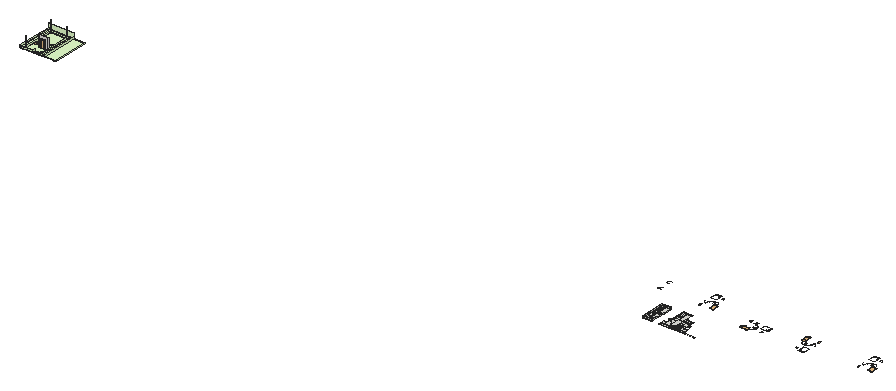
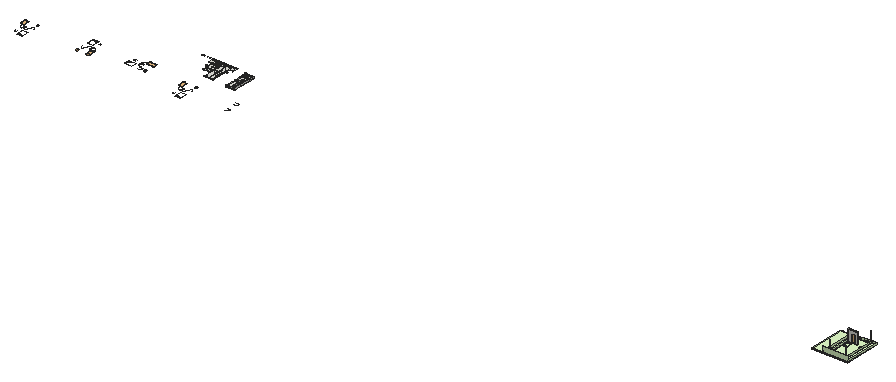
# SketchUp Ruby script. Lengths in inches.
U = 1.inch
M = Sketchup.active_model
def pt(a) = Geom::Point3d.new(a.map { |v| v * U })
def face(e, loops, mat)
  f = e.add_face(loops[0].map { |a| pt(a) })
  loops[1..].each { |l| e.add_face(l.map { |a| pt(a) }).erase! }
  f.material = f.back_material = mat if mat
  f
end
# faces: each face lists its corners as indices into pts; further lists are holes
def faces(e, pts, list, mat = nil) = list.each { |f| face(e, (f[0].is_a?(Array) ? f : [f]).map { |l| l.map { |i| pts[i] } }, mat) }
# xy, xz, yz: faces in a plane at the given z, y or x. An outline is a flat list of corners, or four numbers for a rectangle; further outlines are holes
def ring(l) = l.size == 4 ? [[l[0], l[1]], [l[2], l[1]], [l[2], l[3]], [l[0], l[3]]] : l.each_slice(2).to_a
def flat(e, list, mat, &to3) = list.each { |f| face(e, (f[0].is_a?(Array) ? f : [f]).map { |l| ring(l).map { |u, v| to3.(u, v) } }, mat) }
def xy(e, z, list, mat = nil) = flat(e, list, mat) { |x, y| [x, y, z] }
def xz(e, y, list, mat = nil) = flat(e, list, mat) { |x, z| [x, y, z] }
def yz(e, x, list, mat = nil) = flat(e, list, mat) { |y, z| [x, y, z] }
def lines(e, pts, list) = list.each { |a, b| e.add_line(pt(pts[a]), pt(pts[b])) }
# prism: a flat outline (further loops are holes) pulled along v
def prism(e, loops, v, mat = nil)
  f = face(e, loops, mat); d = Geom::Vector3d.new(v.map { |x| x * U })
  f.pushpull(f.normal.samedirection?(d) ? d.length : -d.length)
end
def box(e, o, s, mat = nil) = prism(e, [[o, [o[0] + s[0], o[1], o[2]], [o[0] + s[0], o[1] + s[1], o[2]], [o[0], o[1] + s[1], o[2]]]], [0, 0, s[2]], mat)
def at(x, y, z, deg = 0) = Geom::Transformation.translation(pt([x, y, z])) * Geom::Transformation.rotation(ORIGIN, Z_AXIS, deg.degrees)
def axes(o, x, y, z) = Geom::Transformation.new([*x, 0, *y, 0, *z, 0, *pt(o).to_a, 1])
def part(name) = M.definitions.add(name)
# library, detail: a bought-in or finely detailed component or shape, given as its bounding box
def library(name, o, s) = part(name).tap { |d| box(d.entities, o, s) }
def detail(e, o, s) = box(e.add_group.entities, o, s)
def put(e, d, t, mat = nil) = e.add_instance(d, t).tap { |i| i.material = mat if mat }
def group(e, t, mat = nil) = e.add_group.tap { |g| g.transformation = t; g.material = mat if mat }.entities
root = M.entities
M.materials.add("[Color F01]").color = [229, 255, 204]
M.materials.add("[Wood Cherry Original]").color = [152, 86, 42]
c1 = part("*U16\#1")
p = [[-20,-17,0],[-20,23,0],[-18.25,23,0],[-18.25,-17,0],[20,-17,0],[19.92,-14.49,0],
  [19.68,-11.99,0],[19.29,-9.5,0],[18.74,-7.05,0],[18.04,-4.64,0],[17.19,-2.28,0],[16.19,0.03,0],
  [15.05,2.27,0],[13.77,4.43,0],[12.36,6.51,0],[10.82,8.5,0],[9.16,10.38,0],[7.38,12.16,0],
  [5.5,13.82,0],[3.51,15.36,0],[1.43,16.77,0],[-0.73,18.05,0],[-2.97,19.19,0],[-5.28,20.19,0],
  [-7.64,21.04,0],[-10.05,21.74,0],[-12.5,22.29,0],[-14.99,22.68,0],[-17.49,22.92,0],[-20,-23,0],
  [20,-23,0]]
lines(c1.entities,p,[[0,1],[1,2],[2,3],[3,0],[4,5],[5,6],[6,7],[7,8],[8,9],[9,10],[10,11],[11,12],
  [12,13],[13,14],[14,15],[15,16],[16,17],[17,18],[18,19],[19,20],[20,21],[21,22],[22,23],[23,24],
  [24,25],[25,26],[26,27],[27,28],[28,1],[0,29],[4,30]])
c2 = part("Bed - Queen\#1")
p = [[22,23.6,0],[16.8,23.6,0],[22,38.8,0],[1.2,38.8,0],[1.2,25.6,0],[-1.2,38.8,0],
  [-1.2,25.6,0],[-22,38.8,0],[-22,25.6,0],[30,-40,0],[-30,-40,0],[-30,40,0],
  [14.8,23.2,0],[-30,23.2,0],[-30,25.6,0],[14.8,25.6,0],[30,40,0],[30,10.4,0],
  [14.8,10.4,0]]
lines(c2.entities,p,[[0,1],[2,0],[3,2],[4,3],[5,6],[7,5],[8,7],[9,10],[10,11],[12,13],[14,15],[11,16],
  [16,9],[17,15],[18,17],[15,18]])
c3 = library("Dining Set - 36 x 72 in.\#1",[-45.5,-27.5,0],[91,55,0.01])
c4 = library("*U20\#1",[-21.75,-46.5,0],[21,33,0.01])
c5 = part("Bed - Queen\#2")
p = [[22,23.6,0],[16.8,23.6,0],[22,38.8,0],[1.2,38.8,0],[1.2,25.6,0],[-1.2,38.8,0],
  [-1.2,25.6,0],[-22,38.8,0],[-22,25.6,0],[30,-40,0],[-30,-40,0],[-30,40,0],
  [14.8,23.2,0],[-30,23.2,0],[-30,25.6,0],[14.8,25.6,0],[30,40,0],[30,10.4,0],
  [14.8,10.4,0]]
lines(c5.entities,p,[[0,1],[2,0],[3,2],[4,3],[5,6],[7,5],[8,7],[9,10],[10,11],[12,13],[14,15],[11,16],
  [16,9],[17,15],[18,17],[15,18]])
c6 = part("*U16\#2")
p = [[-20,-17,0],[-20,23,0],[-18.25,23,0],[-18.25,-17,0],[20,-17,0],[19.92,-14.49,0],
  [19.68,-11.99,0],[19.29,-9.5,0],[18.74,-7.05,0],[18.04,-4.64,0],[17.19,-2.28,0],[16.19,0.03,0],
  [15.05,2.27,0],[13.77,4.43,0],[12.36,6.51,0],[10.82,8.5,0],[9.16,10.38,0],[7.38,12.16,0],
  [5.5,13.82,0],[3.51,15.36,0],[1.43,16.77,0],[-0.73,18.05,0],[-2.97,19.19,0],[-5.28,20.19,0],
  [-7.64,21.04,0],[-10.05,21.74,0],[-12.5,22.29,0],[-14.99,22.68,0],[-17.49,22.92,0],[-20,-23,0],
  [20,-23,0]]
lines(c6.entities,p,[[0,1],[1,2],[2,3],[3,0],[4,5],[5,6],[6,7],[7,8],[8,9],[9,10],[10,11],[11,12],
  [12,13],[13,14],[14,15],[15,16],[16,17],[17,18],[18,19],[19,20],[20,21],[21,22],[22,23],[23,24],
  [24,25],[25,26],[26,27],[27,28],[28,1],[0,29],[4,30]])
c7 = library("Dining Set - 36 x 72 in.\#2",[-45.5,-27.5,0],[91,55,0.01])
c8 = library("*U20\#2",[-21.75,-46.5,0],[21,33,0.01])
c9 = part("Group\#16")
xy(c9.entities,0,[[8.74,0,9,0,9,0.26],[140,3.98,140.02,4,140,4],[0,123.84,0.16,124,0,124],[0,335.97,0.03,336,0,336]])
# 113 loose lines left out
c10 = part("Group\#15")
box(c10.entities,[0,0,0],[67,6,6])
c11 = library("Group\#19",[0,0,0],[36,2,84])
c12 = part("Difference")
prism(c12.entities,[[[0,0,0],[29,0,0],[29,0,84],[65,0,84],[65,0,0],[101,0,0],[101,0,120],[0,0,120]]],[0,10,0])
xy(root,0,[[7085,0,7347,3],[7347,0,7464.37,3],[7085,3,7221,21],[7221,3,7288,9],[7288,3,7347,21],
  [7221,9,7288,15],[7221,15,7288,21],[7085,21,7089,63],[7089,21,7125,63],[7125,21,7221,21,7221,27,7129,27,7129,273,7221,273,7221.38,273.02,7221.76,273.1,7221.95,273.15,7222.125,273.22,7222.3,273.3,7222.47,273.39,7222.64,273.49,7222.79,273.6,7223.09,273.84,7223.22,273.98,7223.35,274.13,7223.46,274.28,7223.57,274.44,7223.66,274.61,7223.74,274.79,7223.82,274.96,7223.875,275.15,7223.92,275.33,7223.96,275.52,7223.99,275.71,7224,275.9,7224,276.1,7223.99,276.29,7223.96,276.48,7223.92,276.67,7223.875,276.85,7223.82,277.04,7223.74,277.21,7223.66,277.39,7223.57,277.56,7223.46,277.72,7223.35,277.87,7223.22,278.02,7223.09,278.16,7222.79,278.4,7222.64,278.51,7222.47,278.61,7222.3,278.7,7222.125,278.78,7221.95,278.85,7221.76,278.9,7221.38,278.98,7221,279,7125,279],
  [7221,21,7307,27],[7307,21,7343,63],[7343,21,7347,63],[7129,27,7221,27,7221,85.4,7218,85.4,7218,62.89,7214.08,61.43,7210.07,60.24,7206,59.31,7201.87,58.64,7197.71,58.24,7193.53,58.11,7189.36,58.26,7185.2,58.67,7181.07,59.36,7177,60.3,7173,61.51,7169.6,62.85,7166.28,64.39,7163.07,66.14,7159.97,68.08,7157,70.21,7154.17,72.52,7151.49,75.01,7148.97,77.66,7146.61,80.45,7144.44,83.39,7142.45,86.46,7142.18,86.94,7140.66,89.65,7139.07,92.9375,7137.6875,96.32,7136.52,99.79,7135.57,103.32,7134.88,106.69,7134.84,106.9,7134.33,110.52,7134.05,114.16,7134,117.82,7134,273,7129,273],[[7221,27,7288,85.4],[7256.5,30,7285,82.4],[7239.51,37.02,7239.51,40.7,7224,40.7,7224,82.4,7252.5,82.4,7252.5,42.7,7247.66,42.7,7247.66,37.02]],
  [7288,27,7307,27,7307,147,7305,147,7305,91.16,7304.96,90.87,7304.91,90.58,7304.83,90.29,7304.74,90.01,7304.63,89.73,7304.5,89.46,7304.36,89.2,7304.2,88.95,7304.02,88.72,7303.83,88.49,7303.625,88.27,7303.41,88.07,7303.18,87.89,7302.93,87.72,7302.68,87.5625,7302.42,87.42,7302.14,87.3,7301.87,87.2,7301.58,87.11,7301.29,87.05,7301,87,7289.57,87,7289.33,86.94,7289.21,86.9,7289.09,86.85,7288.87,86.73,7288.77,86.66,7288.67,86.58,7288.4,86.31,7288.33,86.21,7288.26,86.1,7288.14,85.88,7288.02,85.52,7288,85.4],[7256.5,30,7285,30,7285,40.7,7269.49,40.7,7269.49,37.02,7261.34,37.02,7261.34,40.7,7256.5,40.7],[7239.51,37.02,7247.66,75.22],[7261.34,37.02,7269.49,75.22],[7261.34,37.02,7269.49,75.22],
  [7224,40.7,7239.51,42.7],[7256.5,40.7,7261.34,42.7],[7269.49,40.7,7285,42.7],[7224,42.7,7239.51,55.2],[7247.66,42.7,7252.5,55.2],
  [7256.5,42.7,7261.34,55.2],[7269.49,42.7,7285,55.2],[7224,55.2,7239.51,57.2],[7247.66,55.2,7252.5,57.2],[7256.5,55.2,7261.34,57.2],
  [7269.49,55.2,7285,57.2],[7224,57.2,7239.51,69.7],[7247.66,57.2,7252.5,69.7],[7256.5,57.2,7261.34,69.7],[7269.49,57.2,7285,69.7],
  [7193.53,58.11,7197.71,58.24,7201.87,58.64,7206,59.31,7210.07,60.24,7214.08,61.43,7218,62.89,7218,85.4,7221,85.4,7221,147,7177,147,7177,60.3,7181.07,59.36,7185.2,58.67,7189.36,58.26],[7177,60.3,7177,270,7173,270,7173,61.51],[[7173,61.51,7173,270,7170,270,7170,200.6,7146,200.6,7146,270,7134,270,7134,117.82,7134.05,114.16,7134.33,110.52,7134.84,106.9,7134.88,106.69,7135.57,103.32,7136.52,99.79,7137.6875,96.32,7139.07,92.9375,7140.66,89.65,7142.18,86.94,7142.45,86.46,7144.44,83.39,7146.61,80.45,7148.97,77.66,7151.49,75.01,7154.17,72.52,7157,70.21,7159.97,68.08,7163.07,66.14,7166.28,64.39,7169.6,62.85],[7164.9,119.64,7163.62,119.72,7162.35,119.89,7161.09,120.14,7159.85,120.48,7158.63,120.89,7157.45,121.38,7156.3,121.95,7155.1875,122.59,7154.12,123.3,7153.1,124.09,7152.13,124.93,7151.23,125.84,7150.38,126.8,7149.6,127.82,7148.88,128.89,7148.24,130,7147.67,131.15,7147.17,132.33,7146.76,133.55,7146.61,134.08,7146.42,134.79,7146.17,136.05,7146,137.32,7146,197.6,7170,197.6,7170,120.13,7168.74,119.89,7167.47,119.72,7166.1875,119.64]],[7224,69.7,7239.51,71.7],[7247.66,69.7,7252.5,71.7],
  [7256.5,69.7,7261.34,71.7],[7269.49,69.7,7285,71.7],[7224,71.7,7239.51,71.7,7239.51,75.22,7247.66,75.22,7247.66,71.7,7252.5,71.7,7252.5,82.4,7224,82.4],[7256.5,71.7,7261.34,71.7,7261.34,75.22,7269.49,75.22,7269.49,71.7,7285,71.7,7285,82.4,7256.5,82.4],[7221,85.4,7224.97,85.4,7224.97,115,7269,115,7269,85.4,7288,85.4,7288.02,85.52,7288.14,85.88,7288.26,86.1,7288.33,86.21,7288.4,86.31,7288.67,86.58,7288.77,86.66,7288.87,86.73,7289.09,86.85,7289.21,86.9,7289.33,86.94,7289.57,87,7301,87,7301,147,7221,147],
  [7224.97,85.4,7228.97,85.4,7228.97,111,7265,111,7265,85.4,7269,85.4,7269,115,7224.97,115],[7228.97,85.4,7244.98,111],[7244.98,85.4,7248.98,111],[7248.98,85.4,7265,111],[7301,87,7301.29,87.05,7301.58,87.11,7301.87,87.2,7302.14,87.3,7302.42,87.42,7302.68,87.5625,7302.93,87.72,7303.18,87.89,7303.41,88.07,7303.625,88.27,7303.83,88.49,7304.02,88.72,7304.2,88.95,7304.36,89.2,7304.5,89.46,7304.63,89.73,7304.74,90.01,7304.83,90.29,7304.91,90.58,7304.96,90.87,7305,91.16,7305,147,7301,147],
  [7101,111,7125,115],[7307,111,7331,115],[7164.9,119.64,7166.1875,119.64,7167.47,119.72,7168.74,119.89,7170,120.13,7170,197.6,7146,197.6,7146,137.32,7146.17,136.05,7146.42,134.79,7146.61,134.08,7146.76,133.55,7147.17,132.33,7147.67,131.15,7148.24,130,7148.88,128.89,7149.6,127.82,7150.38,126.8,7151.23,125.84,7152.13,124.93,7153.1,124.09,7154.12,123.3,7155.1875,122.59,7156.3,121.95,7157.45,121.38,7158.63,120.89,7159.85,120.48,7161.09,120.14,7162.35,119.89,7163.62,119.72],[7177,147,7221,153],[7221,147,7307,147,7307.38,147.02,7307.76,147.1,7307.95,147.15,7308.125,147.22,7308.3,147.3,7308.47,147.39,7308.64,147.49,7308.79,147.6,7309.09,147.84,7309.22,147.98,7309.35,148.13,7309.46,148.28,7309.57,148.44,7309.66,148.61,7309.74,148.79,7309.82,148.96,7309.875,149.15,7309.92,149.33,7309.96,149.52,7309.99,149.71,7310,149.9,7310,150.1,7309.99,150.29,7309.96,150.48,7309.92,150.67,7309.875,150.85,7309.82,151.04,7309.74,151.21,7309.66,151.39,7309.57,151.56,7309.46,151.72,7309.35,151.87,7309.22,152.02,7309.09,152.16,7308.79,152.4,7308.64,152.51,7308.47,152.61,7308.3,152.7,7308.125,152.78,7307.95,152.85,7307.76,152.9,7307.38,152.98,7307,153,7221,153],
  [7177,153,7221,156],[7221,153,7305,156],[7177,156,7221,270],[7221,156,7305,158],[7221,158,7244.77,189],
  [7244.77,158,7245.77,189],[7245.77,158,7270.55,189],[7270.55,158,7271.55,189],[7271.55,158,7295,189],[7295,158,7305,189],
  [7221,189,7305,191],[7146,200.6,7170,270],[7134,270,7221,273]])
xy(root,0,[[0,344.07,4,730.07],[4,344.07,40,730.07],[40,344.07,144,362.07],[144,344.07,180,348.07],[180,344.07,180,362.07,220,362.07,220,698.07,180,698.07,180,730.07,258,730.07,258,344.07],
  [258,344.07,262,730.07],[262,344.07,379.37,730.07],[144,348.07,180,355.07],[144,355.07,180,362.07],[40,362.07,44,694.07],
  [44,362.07,144,366.07],[144,362.07,180,366.07],[180,362.07,180,366.07,216,366.07,216,698.07,220,698.07,220,362.07],[44,366.07,144,694.07],[144,366.07,180,694.07],
  [180,366.07,216,694.07],[40,694.07,40,730.07,144,730.07,144,698.07,40.03,698.07,40.03,694.07],[40.03,694.07,144,698.07],[144,694.07,180,698.07],[180,694.07,216,698.07],
  [144,698.07,180,730.07]],"[Color F01]")
xy(root,3,[[0,344.07,136,344.07,136,362.07,40,362.07,40,730.07,0,730.07],[136,344.07,203,344.07,203,698.07,40,698.07,40,362.07,136,362.07],[262,344.07,379.37,730.07],[203,362.07,220,698.07],[40,698.07,136,730.07],
  [136,698.07,203,730.07],[203,698.07,220,730.07]],"[Color F01]")
xz(root,344.07,[[0,0,40,3],[40,0,379.37,3],[0,3,40,21],[40,3,136,21],[203,3,262,21]],"[Color F01]")
xz(root,362.07,[[40,0,44,3],[44,0,216,0,216,3,203,3,203,9,136,9,136,3,44,3],[216,0,220,3],[40,3,44,120],[203,3,216,21],
  [216,3,220,21]],"[Color F01]")
xz(root,694.07,[[40.03,0,44,120]],"[Color F01]")
xz(root,698.07,[[40.03,0,216,3],[216,0,220,3],[40,3,40.03,21],[40.03,3,216,21],[216,3,220,21]],"[Color F01]")
xz(root,730.07,[[0,0,379.37,3],[0,3,262,63]],"[Color F01]")
yz(root,0,[[344.07,0,730.07,3],[344.07,3,730.07,21]],"[Color F01]")
yz(root,40,[[362.07,0,694.07,3],[362.07,3,694.07,21],[694.07,3,698.07,21]],"[Color F01]")
yz(root,40.03,[[694.07,0,698.07,120]],"[Color F01]")
yz(root,44,[[362.07,0,366.07,120]],"[Color F01]")
yz(root,136,[[344.07,3,362.07,21]],"[Color F01]")
yz(root,144,[[437.07,3.09,441.07,91.09]])
yz(root,180,[[437.07,3.09,441.07,91.09]])
yz(root,203,[[344.07,3,362.07,9]],"[Color F01]")
yz(root,216,[[694.07,0,698.07,120]],"[Color F01]")
yz(root,220,[[362.07,0,698.07,3],[362.07,3,698.07,21]],"[Color F01]")
yz(root,262,[[344.07,3,730.07,21]],"[Color F01]")
yz(root,379.37,[[362.07,0,730.07,3]],"[Color F01]")
g1 = group(root,at(6896,21,-20))
prism(g1,[[[96,252,0],[96,170,0],[96,168,0],[96,0,0],[0,0,0],[0,42,0],[0,90,0],[0,94,0],[0,258,0],[96,258,0],[96.19,257.99,0],[96.38,257.98,0],[96.57,257.94,0],[96.76,257.9,0],[96.95,257.85,0],[97.125,257.78,0],[97.3,257.7,0],[97.47,257.61,0],[97.64,257.51,0],[97.79,257.4,0],[97.94,257.28,0],[98.09,257.16,0],[98.22,257.02,0],[98.35,256.87,0],[98.46,256.72,0],[98.57,256.56,0],[98.66,256.39,0],[98.74,256.21,0],[98.82,256.04,0],[98.875,255.85,0],[98.92,255.67,0],[98.96,255.48,0],[98.99,255.29,0],[99,255.1,0],[99,254.9,0],[98.99,254.71,0],[98.96,254.52,0],[98.92,254.33,0],[98.875,254.15,0],[98.82,253.96,0],[98.74,253.79,0],[98.66,253.61,0],[98.57,253.44,0],[98.46,253.28,0],[98.35,253.13,0],[98.22,252.98,0],[98.09,252.84,0],[97.94,252.72,0],[97.79,252.6,0],[97.64,252.49,0],[97.47,252.39,0],[97.3,252.3,0],[97.125,252.22,0],[96.95,252.15,0],[96.76,252.1,0],[96.57,252.06,0],[96.38,252.02,0],[96.19,252.01,0]]],[0,0,6])
g2 = group(root,at(6948,147,-14))
box(g2,[0,0,0],[44,6,4])
g3 = group(root,at(6948,153,-14))
box(g3,[0,0,0],[44,3,4])
g4 = group(root,at(6896,21,-14))
xy(g4,0,[[0,0,0,258,96,258,96.38,257.98,96.76,257.9,96.95,257.85,97.125,257.78,97.3,257.7,97.47,257.61,97.64,257.51,97.79,257.4,98.09,257.16,98.22,257.02,98.35,256.87,98.46,256.72,98.57,256.56,98.66,256.39,98.74,256.21,98.82,256.04,98.875,255.85,98.92,255.67,98.96,255.48,98.99,255.29,99,255.1,99,254.9,98.99,254.71,98.96,254.52,98.92,254.33,98.875,254.15,98.82,253.96,98.74,253.79,98.66,253.61,98.57,253.44,98.46,253.28,98.35,253.13,98.22,252.98,98.09,252.84,97.79,252.6,97.64,252.49,97.47,252.39,97.3,252.3,97.125,252.22,96.95,252.15,96.76,252.1,96.38,252.02,96,252,4,252,4,6,96,6,96,0]])
g5 = group(g4,at(1095,0,0))
g6 = group(g5,at(-1095,0,0))
xy(g6,14,[[0,0,96,0,96,6,4,6,4,252,96,252,96.38,252.02,96.76,252.1,96.95,252.15,97.125,252.22,97.3,252.3,97.47,252.39,97.64,252.49,97.79,252.6,98.09,252.84,98.22,252.98,98.35,253.13,98.46,253.28,98.57,253.44,98.66,253.61,98.74,253.79,98.82,253.96,98.875,254.15,98.92,254.33,98.96,254.52,98.99,254.71,99,254.9,99,255.1,98.99,255.29,98.96,255.48,98.92,255.67,98.875,255.85,98.82,256.04,98.74,256.21,98.66,256.39,98.57,256.56,98.46,256.72,98.35,256.87,98.22,257.02,98.09,257.16,97.79,257.4,97.64,257.51,97.47,257.61,97.3,257.7,97.125,257.78,96.95,257.85,96.76,257.9,96.38,257.98,96,258,0,258]])
xz(g6,0,[[0,0,96,14]])
xz(g6,6,[[4,0,96,14]])
xz(g6,252,[[4,0,96,14]])
xz(g6,258,[[0,0,96,14]])
yz(g6,0,[[0,0,258,14]])
yz(g6,4,[[6,0,252,14]])
yz(g6,96,[[0,0,6,14]])
yz(g6,99,[[254.9,0,255.1,14]])
p = [[96,252,0],[96.19,252.01,0],[96.19,252.01,14],[96,252,14],[96.38,252.02,0],[96.38,252.02,14],
  [96.57,252.06,0],[96.57,252.06,14],[96.76,252.1,0],[96.76,252.1,14],[96.95,252.15,0],[96.95,252.15,14],
  [97.125,252.22,0],[97.125,252.22,14],[97.3,252.3,0],[97.3,252.3,14],[97.47,252.39,0],[97.47,252.39,14],
  [97.64,252.49,0],[97.64,252.49,14],[97.79,252.6,0],[97.79,252.6,14],[97.94,252.72,0],[97.94,252.72,14],
  [98.09,252.84,0],[98.09,252.84,14],[98.22,252.98,0],[98.22,252.98,14],[98.35,253.13,0],[98.35,253.13,14],
  [98.46,253.28,0],[98.46,253.28,14],[98.57,253.44,0],[98.57,253.44,14],[98.66,253.61,0],[98.66,253.61,14],
  [98.74,253.79,0],[98.74,253.79,14],[98.82,253.96,0],[98.82,253.96,14],[98.875,254.15,0],[98.875,254.15,14],
  [98.92,254.33,0],[98.92,254.33,14],[98.96,254.52,0],[98.96,254.52,14],[98.99,254.71,0],[98.99,254.71,14],
  [99,254.9,0],[99,254.9,14],[99,255.1,0],[98.99,255.29,0],[98.99,255.29,14],[99,255.1,14],
  [98.96,255.48,0],[98.96,255.48,14],[98.92,255.67,0],[98.92,255.67,14],[98.875,255.85,0],[98.875,255.85,14],
  [98.82,256.04,0],[98.82,256.04,14],[98.74,256.21,0],[98.74,256.21,14],[98.66,256.39,0],[98.66,256.39,14],
  [98.57,256.56,0],[98.57,256.56,14],[98.46,256.72,0],[98.46,256.72,14],[98.35,256.87,0],[98.35,256.87,14],
  [98.22,257.02,0],[98.22,257.02,14],[98.09,257.16,0],[98.09,257.16,14],[97.94,257.28,0],[97.94,257.28,14],
  [97.79,257.4,0],[97.79,257.4,14],[97.64,257.51,0],[97.64,257.51,14],[97.47,257.61,0],[97.47,257.61,14],
  [97.3,257.7,0],[97.3,257.7,14],[97.125,257.78,0],[97.125,257.78,14],[96.95,257.85,0],[96.76,257.9,0],
  [96.76,257.9,14],[96.95,257.85,14],[96.57,257.94,0],[96.38,257.98,0],[96.38,257.98,14],[96.57,257.94,14],
  [96.19,257.99,0],[96,258,0],[96,258,14],[96.19,257.99,14]]
faces(g6,p,[[0,1,2,3],[1,4,5,2],[4,6,7,5],[6,8,9,7],[8,10,11,9],[10,12,13,11],[12,14,15,13],[14,16,17,15],
  [16,18,19,17],[18,20,21,19],[20,22,23,21],[22,24,25,23],[24,26,27,25],[26,28,29,27],[28,30,31,29],[30,32,33,31],
  [32,34,35,33],[34,36,37,35],[36,38,39,37],[38,40,41,39],[40,42,43,41],[42,44,45,43],[44,46,47,45],[46,48,49,47],
  [50,51,52,53],[51,54,55,52],[54,56,57,55],[56,58,59,57],[58,60,61,59],[60,62,63,61],[62,64,65,63],[64,66,67,65],
  [66,68,69,67],[68,70,71,69],[70,72,73,71],[72,74,75,73],[74,76,77,75],[76,78,79,77],[78,80,81,79],[80,82,83,81],
  [82,84,85,83],[84,86,87,85],[88,89,90,91],[86,88,91,87],[92,93,94,95],[89,92,95,90],[96,97,98,99],[93,96,99,94]])
g7 = group(root,at(6913.91,116.63,-14))
xy(g7,0,[[[22.92,0,24.38,0.0625,25.84,0.22,27.27,0.47,28.69,0.82,30.09,1.25,30.09,156.37,0.09,156.37,0.09,24.79,0,23.33,0,21.87,0.1,20.41,0.29,18.96,0.58,17.53,0.96,16.12,1.42,14.73,1.98,13.38,2.62,12.07,3.09,11.25,3.34,10.8,3.7,10.25,4.15,9.58,5.03,8.41,5.99,7.31,7.01,6.27,8.1,5.29,9.25,4.39,10.45,3.5625,11.71,2.82,13.01,2.15,14.35,1.57,15.73,1.08,17.13,0.68,18.5625,0.37,20.01,0.15,21.46,0.03],[21.99,3.01,20.71,3.09,19.4375,3.26,18.18,3.51,16.94,3.85,15.72,4.26,14.54,4.75,13.39,5.32,12.28,5.96,11.21,6.67,10.1875,7.46,9.22,8.3,8.32,9.21,7.47,10.17,6.69,11.19,5.97,12.26,5.33,13.37,4.76,14.52,4.26,15.7,3.85,16.92,3.7,17.45,3.51,18.16,3.26,19.42,3.09,20.6875,3.09,80.97,27.09,80.97,27.09,3.5,25.83,3.26,24.56,3.09,23.28,3.01],[3.09,83.97,27.09,153.37]]])
xz(g7,80.97,[[3.09,0,27.09,1],[3.09,1,27.09,2]])
xz(g7,83.97,[[3.09,0,27.09,2]])
xz(g7,153.37,[[3.09,0,27.09,2]])
xz(g7,156.37,[[0.09,0,30.09,2]])
yz(g7,0,[[21.87,0,23.33,2]])
yz(g7,0.09,[[24.79,0,153.37,2],[153.37,0,156.37,2]])
yz(g7,3.09,[[20.6875,0,80.97,2],[83.97,0,153.37,2]])
yz(g7,27.09,[[3.5,0,80.97,1],[83.97,0,153.37,2],[3.5,1,80.97,2]])
yz(g7,30.09,[[1.25,0,153.37,2],[153.37,0,156.37,2]])
p = [[20.01,0.15,0],[21.46,0.03,0],[21.46,0.03,2],[20.01,0.15,2],[22.92,0,0],[22.92,0,2],
  [24.38,0.0625,0],[24.38,0.0625,2],[25.84,0.22,0],[25.84,0.22,2],[18.5625,0.37,0],[18.5625,0.37,2],
  [27.27,0.47,0],[27.27,0.47,2],[17.13,0.68,0],[17.13,0.68,2],[28.69,0.82,0],[28.69,0.82,2],
  [15.73,1.08,0],[15.73,1.08,2],[30.09,1.25,0],[30.09,1.25,2],[14.35,1.57,0],[14.35,1.57,2],
  [13.01,2.15,0],[13.01,2.15,2],[11.71,2.82,0],[11.71,2.82,2],[10.45,3.5625,0],[10.45,3.5625,2],
  [9.25,4.39,0],[9.25,4.39,2],[8.1,5.29,0],[8.1,5.29,2],[7.01,6.27,0],[7.01,6.27,2],
  [5.99,7.31,0],[5.99,7.31,2],[5.03,8.41,0],[5.03,8.41,2],[4.15,9.58,0],[4.15,9.58,2],
  [3.7,10.25,0],[3.7,10.25,2],[3.34,10.8,0],[3.34,10.8,2],[3.09,11.25,0],[3.09,11.25,2],
  [2.62,12.07,0],[2.62,12.07,2],[1.98,13.38,0],[1.98,13.38,2],[1.42,14.73,0],[1.42,14.73,2],
  [0.96,16.12,0],[0.96,16.12,2],[0.58,17.53,0],[0.58,17.53,2],[0.29,18.96,0],[0.29,18.96,2],
  [0.1,20.41,0],[0.1,20.41,2],[0,21.87,0],[0,21.87,2],[0.09,24.79,0],[0,23.33,0],
  [0,23.33,2],[0.09,24.79,2]]
faces(g7,p,[[0,1,2,3],[1,4,5,2],[4,6,7,5],[6,8,9,7],[10,0,3,11],[8,12,13,9],[14,10,11,15],[12,16,17,13],
  [18,14,15,19],[16,20,21,17],[22,18,19,23],[24,22,23,25],[26,24,25,27],[28,26,27,29],[30,28,29,31],[32,30,31,33],
  [34,32,33,35],[36,34,35,37],[38,36,37,39],[40,38,39,41],[42,40,41,43],[44,42,43,45],[46,44,45,47],[48,46,47,49],
  [50,48,49,51],[52,50,51,53],[54,52,53,55],[56,54,55,57],[58,56,57,59],[60,58,59,61],[62,60,61,63],[64,65,66,67]])
g8 = group(g7,at(0,0,2))
xy(g8,0,[[[22.92,0,24.38,0.0625,25.84,0.22,27.27,0.47,28.69,0.82,30.09,1.25,30.09,156.37,0.09,156.37,0.09,24.79,0,23.33,0,21.87,0.1,20.41,0.29,18.96,0.58,17.53,0.96,16.12,1.42,14.73,1.98,13.38,2.62,12.07,3.09,11.25,3.34,10.8,3.7,10.25,4.15,9.58,5.03,8.41,5.99,7.31,7.01,6.27,8.1,5.29,9.25,4.39,10.45,3.5625,11.71,2.82,13.01,2.15,14.35,1.57,15.73,1.08,17.13,0.68,18.5625,0.37,20.01,0.15,21.46,0.03],[21.99,3.01,20.71,3.09,19.4375,3.26,18.18,3.51,16.94,3.85,15.72,4.26,14.54,4.75,13.39,5.32,12.28,5.96,11.21,6.67,10.1875,7.46,9.22,8.3,8.32,9.21,7.47,10.17,6.69,11.19,5.97,12.26,5.33,13.37,4.76,14.52,4.26,15.7,3.85,16.92,3.7,17.45,3.51,18.16,3.26,19.42,3.09,20.6875,3.09,80.97,27.09,80.97,27.09,3.5,25.83,3.26,24.56,3.09,23.28,3.01],[3.09,83.97,27.09,153.37]]])
g9 = group(root,at(6944,60.3,-14))
prism(g9,[[[0,57.58,0],[0,209.7,0],[4,209.7,0],[4,95.7,0],[4,92.7,0],[4,86.7,0],[4,0,0],[0,1.21,0]]],[0,0,2])
g10 = group(root,at(6900,27,-14))
prism(g10,[[[48,33.3,0],[52.07,32.36,0],[56.2,31.67,0],[60.36,31.26,0],[64.53,31.11,0],[68.71,31.24,0],[72.87,31.64,0],[77,32.31,0],[81.07,33.24,0],[85.08,34.43,0],[89,35.89,0],[89,58.4,0],[92,58.4,0],[92,0,0],[0,0,0],[0,246,0],[5,246,0],[5,243,0],[5,90.82,0],[5.05,87.16,0],[5.33,83.52,0],[5.84,79.9,0],[6.57,76.32,0],[7.52,72.79,0],[8.6875,69.32,0],[10.07,65.9375,0],[11.66,62.65,0],[13.18,59.94,0],[13.45,59.46,0],[15.44,56.39,0],[17.61,53.45,0],[19.97,50.66,0],[22.49,48.01,0],[25.17,45.52,0],[28,43.21,0],[30.97,41.08,0],[34.07,39.14,0],[37.28,37.39,0],[40.6,35.85,0],[44,34.51,0]]],[0,0,6])
g11 = group(root,at(6905,61.51,-14))
prism(g11,[[[0,56.3,0],[0,211.49,0],[9,211.49,0],[9,79.9,0],[8.91,78.45,0],[8.91,76.98,0],[9.01,75.53,0],[9.2,74.08,0],[9.49,72.64,0],[9.87,71.23,0],[10.33,69.85,0],[10.89,68.5,0],[11.53,67.18,0],[12.25,65.91,0],[12.61,65.37,0],[13.06,64.7,0],[13.94,63.53,0],[14.9,62.42,0],[15.92,61.38,0],[17.01,60.41,0],[18.16,59.51,0],[19.36,58.68,0],[20.62,57.93,0],[21.92,57.27,0],[23.26,56.69,0],[24.64,56.2,0],[26.04,55.8,0],[27.47,55.49,0],[28.92,55.27,0],[30.37,55.14,0],[31.83,55.11,0],[33.29,55.18,0],[34.75,55.34,0],[36.18,55.59,0],[37.6,55.93,0],[39,56.37,0],[39,0,0],[35.6,1.33,0],[32.28,2.875,0],[29.07,4.625,0],[25.97,6.57,0],[23,8.7,0],[20.17,11.01,0],[17.49,13.49,0],[14.97,16.14,0],[12.61,18.9375,0],[10.44,21.88,0],[8.45,24.95,0],[8.18,25.43,0],[6.66,28.13,0],[5.07,31.42,0],[3.6875,34.81,0],[2.52,38.27,0],[1.57,41.8,0],[0.84,45.38,0],[0.33,49,0],[0.05,52.65,0]]],[0,0,3])
put(root,c1,axes([7202.01,566.76,0],[-0.89959,0,0],[0,0.89959,0],[0,0,0.89959]))
put(root,c1,axes([7251.98,566.75,0],[0.89894,0,0],[0,0.89894,0],[0,0,0.89894]))
put(root,c1,axes([7157,532.83,0],[-0.74985,0,0],[0,-0.74985,0],[0,0,0.74985]))
put(root,c1,axes([7244.99,658.71,0],[0.54953,0,0],[0,0.54953,0],[0,0,0.54953]))
put(root,c2,at(7175.23,654.07,0))
put(root,c3,axes([7272.51,499.72,0],[0,-0.72425,0],[0.72425,0,0],[0,0,0.72425]))
put(root,c4,axes([7147.22,453.7,0],[-0.62047,0,0],[0,-0.62047,0],[0,0,0.62047]))
put(root,c1,axes([7753.71,465.0625,0],[0,0.89959,0],[0.89959,0,0],[0,0,0.89959]))
put(root,c1,axes([7753.69,415.09,0],[0,-0.89894,0],[0.89894,0,0],[0,0,0.89894]))
put(root,c1,axes([7719.77,510.07,0],[0,0.74985,0],[-0.74985,0,0],[0,0,0.74985]))
put(root,c1,axes([7845.65,422.08,0],[0,-0.54953,0],[0.54953,0,0],[0,0,0.54953]))
put(root,c2,at(7841.02,491.84,0,-90))
put(root,c3,axes([7686.67,394.56,0],[-0.72425,0,0],[0,-0.72425,0],[0,0,0.72425]))
put(root,c4,axes([7640.64,519.86,0],[0,0.62047,0],[-0.62047,0,0],[0,0,0.62047]))
put(root,c1,axes([8278.42,493.38,0],[0.89959,0,0],[0,-0.89959,0],[0,0,0.89959]))
put(root,c1,axes([8228.45,493.4,0],[-0.89894,0,0],[0,-0.89894,0],[0,0,0.89894]))
put(root,c1,axes([8323.43,527.32,0],[0.74985,0,0],[0,0.74985,0],[0,0,0.74985]))
put(root,c1,axes([8235.44,401.43,0],[-0.54953,0,0],[0,-0.54953,0],[0,0,0.54953]))
put(root,c2,at(8305.2,406.07,0,180))
put(root,c3,axes([8207.92,560.42,0],[0,0.72425,0],[-0.72425,0,0],[0,0,0.72425]))
put(root,c4,axes([8333.22,606.45,0],[0.62047,0,0],[0,0.62047,0],[0,0,0.62047]))
put(root,c1,axes([8889.05,566.76,0],[-0.89959,0,0],[0,0.89959,0],[0,0,0.89959]))
put(root,c1,axes([8939.02,566.75,0],[0.89894,0,0],[0,0.89894,0],[0,0,0.89894]))
put(root,c1,axes([8844.04,532.83,0],[-0.74985,0,0],[0,-0.74985,0],[0,0,0.74985]))
put(root,c1,axes([8932.03,658.71,0],[0.54953,0,0],[0,0.54953,0],[0,0,0.54953]))
put(root,c2,at(8862.27,654.07,0))
put(root,c3,axes([8959.55,499.72,0],[0,-0.72425,0],[0.72425,0,0],[0,0,0.72425]))
put(root,c4,axes([8834.25,453.7,0],[-0.62047,0,0],[0,-0.62047,0],[0,0,0.62047]))
put(root,c1,axes([6713.29,603.0625,0],[0,0.89959,0],[-0.89959,0,0],[0,0,0.89959]))
put(root,c1,axes([6713.29,485.0625,0],[0,0.89959,0],[-0.89959,0,0],[0,0,0.89959]))
put(root,c1,axes([8895.35,1087.71,0],[0,0.89959,0],[-0.89959,0,0],[0,0,0.89959]))
put(root,c1,axes([8895.35,969.71,0],[0,0.89959,0],[-0.89959,0,0],[0,0,0.89959]))
put(root,c5,at(90.23,654.07,0))
put(root,c6,axes([72,532.83,0],[-0.74985,0,0],[0,-0.74985,0],[0,0,0.74985]))
put(root,c6,axes([159.99,658.71,0],[0.54953,0,0],[0,0.54953,0],[0,0,0.54953]))
put(root,c6,axes([166.98,566.75,0],[0.89894,0,0],[0,0.89894,0],[0,0,0.89894]))
put(root,c6,axes([117.01,566.76,0],[-0.89959,0,0],[0,0.89959,0],[0,0,0.89959]))
put(root,c7,axes([187.51,499.72,0],[0,-0.72425,0],[0.72425,0,0],[0,0,0.72425]))
put(root,c8,axes([62.22,453.7,0],[-0.62047,0,0],[0,-0.62047,0],[0,0,0.62047]))
put(root,c9,at(40,362.07,0))
put(root,c10,axes([135.95,344.07,3],[1,0,0],[0,0,1],[0,-1,0]),"[Wood Cherry Original]")
g12 = group(root,at(140,437.07,3.09))
xy(g12,84,[[4,0,40,4]])
xy(g12,88,[[0,0,44,4]])
xz(g12,0,[[0,0,4,88],[40,0,44,0,44,88,4,88,4,84,40,84]])
xz(g12,4,[[0,0,4,0,4,84,40,84,40,0,44,0,44,88,0,88]])
yz(g12,0,[[0,0,4,88]])
yz(g12,4,[[0,0,3.33,84],[3.33,0,4,84]])
yz(g12,40,[[0,0,2.21,84],[2.21,0,3.98,84],[3.98,0,4,84]])
yz(g12,44,[[0,0,4,88]])
put(root,c11,at(144,437.07,3.09))
put(root,c12,at(115,441.07,3.09))
